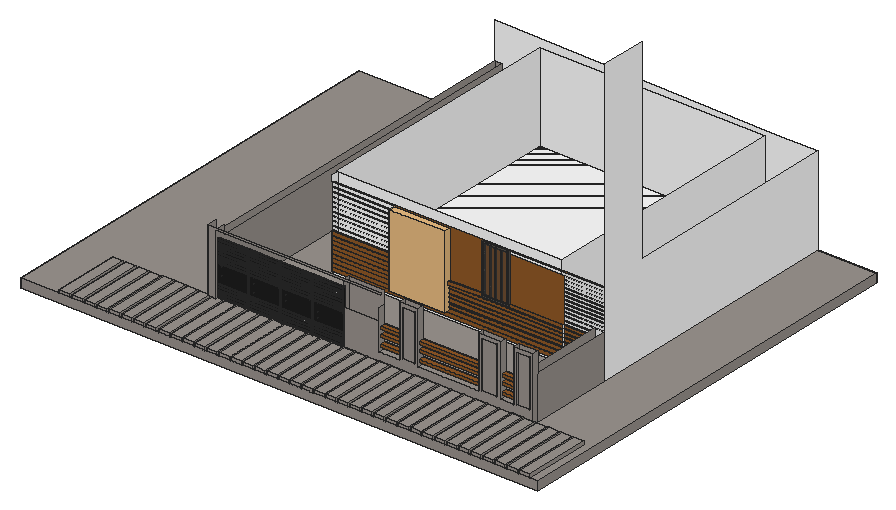
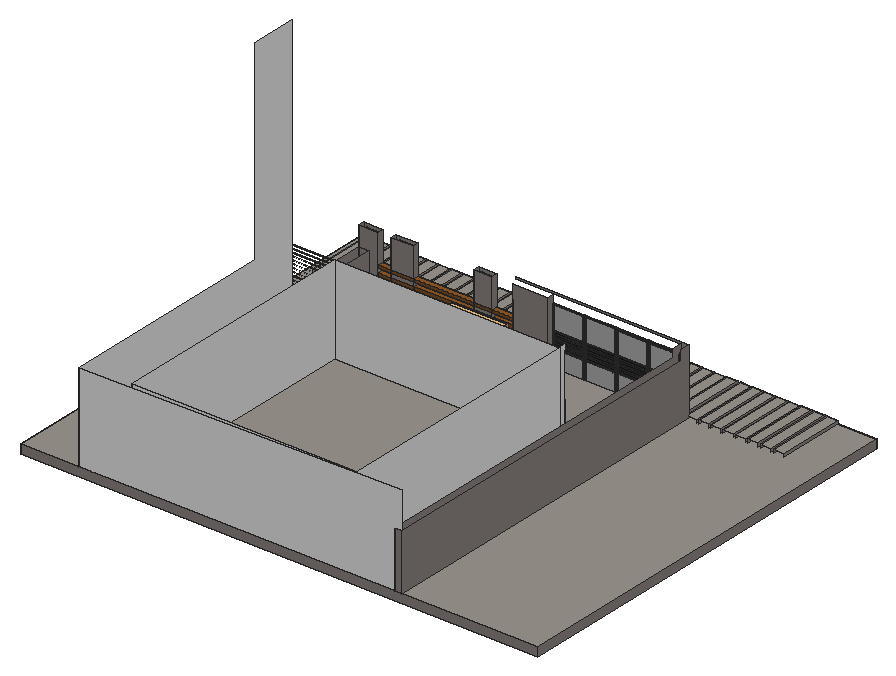
# SketchUp Ruby script. Lengths in inches.
U = 1.inch
M = Sketchup.active_model
def pt(a) = Geom::Point3d.new(a.map { |v| v * U })
def face(e, loops, mat)
  f = e.add_face(loops[0].map { |a| pt(a) })
  loops[1..].each { |l| e.add_face(l.map { |a| pt(a) }).erase! }
  f.material = f.back_material = mat if mat
  f
end
# faces: each face lists its corners as indices into pts; further lists are holes
def faces(e, pts, list, mat = nil) = list.each { |f| face(e, (f[0].is_a?(Array) ? f : [f]).map { |l| l.map { |i| pts[i] } }, mat) }
# xy, xz, yz: faces in a plane at the given z, y or x. An outline is a flat list of corners, or four numbers for a rectangle; further outlines are holes
def ring(l) = l.size == 4 ? [[l[0], l[1]], [l[2], l[1]], [l[2], l[3]], [l[0], l[3]]] : l.each_slice(2).to_a
def flat(e, list, mat, &to3) = list.each { |f| face(e, (f[0].is_a?(Array) ? f : [f]).map { |l| ring(l).map { |u, v| to3.(u, v) } }, mat) }
def xy(e, z, list, mat = nil) = flat(e, list, mat) { |x, y| [x, y, z] }
def xz(e, y, list, mat = nil) = flat(e, list, mat) { |x, z| [x, y, z] }
def yz(e, x, list, mat = nil) = flat(e, list, mat) { |y, z| [x, y, z] }
def lines(e, pts, list) = list.each { |a, b| e.add_line(pt(pts[a]), pt(pts[b])) }
# prism: a flat outline (further loops are holes) pulled along v
def prism(e, loops, v, mat = nil)
  f = face(e, loops, mat); d = Geom::Vector3d.new(v.map { |x| x * U })
  f.pushpull(f.normal.samedirection?(d) ? d.length : -d.length)
end
def box(e, o, s, mat = nil) = prism(e, [[o, [o[0] + s[0], o[1], o[2]], [o[0] + s[0], o[1] + s[1], o[2]], [o[0], o[1] + s[1], o[2]]]], [0, 0, s[2]], mat)
def at(x, y, z, deg = 0) = Geom::Transformation.translation(pt([x, y, z])) * Geom::Transformation.rotation(ORIGIN, Z_AXIS, deg.degrees)
def axes(o, x, y, z) = Geom::Transformation.new([*x, 0, *y, 0, *z, 0, *pt(o).to_a, 1])
def part(name) = M.definitions.add(name)
# library, detail: a bought-in or finely detailed component or shape, given as its bounding box
def library(name, o, s) = part(name).tap { |d| box(d.entities, o, s) }
def detail(e, o, s) = box(e.add_group.entities, o, s)
def put(e, d, t, mat = nil) = e.add_instance(d, t).tap { |i| i.material = mat if mat }
def group(e, t, mat = nil) = e.add_group.tap { |g| g.transformation = t; g.material = mat if mat }.entities
root = M.entities
M.materials.add("Aluminum_Anodized_DarkGray").color = [87, 83, 78]
M.materials.add("Color_008").color = [30, 30, 30]
M.materials.add("Glass_Coated_Black").color = [65, 65, 65]
M.materials["Glass_Coated_Black"].alpha = 0.42
M.materials.add("[0055_LightGoldenrodYellow]").color = [250, 250, 210]
M.materials.add("[0131_Silver]").color = [192, 192, 192]
M.materials.add("[0134_DimGray]").color = [105, 105, 105]
M.materials.add("[Color M00]").color = [255, 255, 255]
M.materials.add("[Granite Tile]").color = [155, 148, 143]
M.materials.add("[Wood Floor Parquet]").color = [145, 89, 39]
c1 = part("Gate slat")
box(c1.entities,[0,0,-2.03],[1.97,0.97,40.94])
c2 = part("Gate frame member")
box(c2.entities,[0,0,0],[1.9,0.97,93.54])
c3 = part("Gate slat \#1")
box(c3.entities,[2.95,0,-2.03],[0.99,0.97,40.94])
c4 = part("Slatted gate leaf")
p = [[42.85,0.97,43.31],[42.85,0.97,44.29]]
lines(c4.entities,p,[[0,1]])
put(c4.entities,c1,axes([3.9375,0,86.61],[0,0,-1],[0,1,0],[1,0,0]),"Color_008")
put(c4.entities,c2,axes([87.6,0,0],[1,0,0],[0,1,0],[0,0,0.92593]),"Color_008")
put(c4.entities,c1,axes([48.6875,0,86.61],[0,0,-1],[0,1,0],[1,0,0]),"Color_008")
put(c4.entities,c2,axes([0,0,0],[1,0,0],[0,1,0],[0,0,0.92593]),"Color_008")
put(c4.entities,c2,axes([42.85,0,0],[1,0,0],[0,1,0],[0,0,0.92593]),"Color_008")
put(c4.entities,c2,axes([44.75,0,0],[1,0,0],[0,1,0],[0,0,0.92593]),"Color_008")
put(c4.entities,c3,axes([3.9375,0,87.11],[0,0,-1],[0,1,0],[1,0,0]),"[0134_DimGray]")
put(c4.entities,c3,axes([48.6875,0,87.11],[0,0,-1],[0,1,0],[1,0,0]),"[0134_DimGray]")
put(c4.entities,c1,axes([48.6875,0,82.68],[0,0,-1],[0,1,0],[1,0,0]),"Color_008")
put(c4.entities,c3,axes([48.6875,0,83.17],[0,0,-1],[0,1,0],[1,0,0]),"[0134_DimGray]")
put(c4.entities,c3,axes([3.9375,0,83.17],[0,0,-1],[0,1,0],[1,0,0]),"[0134_DimGray]")
put(c4.entities,c1,axes([3.9375,0,82.68],[0,0,-1],[0,1,0],[1,0,0]),"Color_008")
put(c4.entities,c3,axes([48.6875,0,75.3],[0,0,-1],[0,1,0],[1,0,0]),"[0134_DimGray]")
put(c4.entities,c1,axes([48.6875,0,78.74],[0,0,-1],[0,1,0],[1,0,0]),"Color_008")
put(c4.entities,c1,axes([48.6875,0,74.8],[0,0,-1],[0,1,0],[1,0,0]),"Color_008")
put(c4.entities,c3,axes([48.6875,0,79.23],[0,0,-1],[0,1,0],[1,0,0]),"[0134_DimGray]")
put(c4.entities,c3,axes([3.9375,0,75.3],[0,0,-1],[0,1,0],[1,0,0]),"[0134_DimGray]")
put(c4.entities,c1,axes([3.9375,0,78.74],[0,0,-1],[0,1,0],[1,0,0]),"Color_008")
put(c4.entities,c3,axes([3.9375,0,79.23],[0,0,-1],[0,1,0],[1,0,0]),"[0134_DimGray]")
put(c4.entities,c1,axes([3.9375,0,74.8],[0,0,-1],[0,1,0],[1,0,0]),"Color_008")
put(c4.entities,c3,axes([48.6875,0,67.42],[0,0,-1],[0,1,0],[1,0,0]),"[0134_DimGray]")
put(c4.entities,c3,axes([3.9375,0,63.48],[0,0,-1],[0,1,0],[1,0,0]),"[0134_DimGray]")
put(c4.entities,c3,axes([48.6875,0,71.36],[0,0,-1],[0,1,0],[1,0,0]),"[0134_DimGray]")
put(c4.entities,c3,axes([3.9375,0,67.42],[0,0,-1],[0,1,0],[1,0,0]),"[0134_DimGray]")
put(c4.entities,c1,axes([3.9375,0,70.87],[0,0,-1],[0,1,0],[1,0,0]),"Color_008")
put(c4.entities,c1,axes([48.6875,0,70.87],[0,0,-1],[0,1,0],[1,0,0]),"Color_008")
put(c4.entities,c1,axes([48.6875,0,66.93],[0,0,-1],[0,1,0],[1,0,0]),"Color_008")
put(c4.entities,c1,axes([48.6875,0,59.06],[0,0,-1],[0,1,0],[1,0,0]),"Color_008")
put(c4.entities,c1,axes([3.9375,0,55.12],[0,0,-1],[0,1,0],[1,0,0]),"Color_008")
put(c4.entities,c1,axes([3.9375,0,62.99],[0,0,-1],[0,1,0],[1,0,0]),"Color_008")
put(c4.entities,c3,axes([3.9375,0,59.55],[0,0,-1],[0,1,0],[1,0,0]),"[0134_DimGray]")
put(c4.entities,c1,axes([3.9375,0,66.93],[0,0,-1],[0,1,0],[1,0,0]),"Color_008")
put(c4.entities,c1,axes([48.6875,0,62.99],[0,0,-1],[0,1,0],[1,0,0]),"Color_008")
put(c4.entities,c3,axes([48.6875,0,59.55],[0,0,-1],[0,1,0],[1,0,0]),"[0134_DimGray]")
put(c4.entities,c3,axes([48.6875,0,63.48],[0,0,-1],[0,1,0],[1,0,0]),"[0134_DimGray]")
put(c4.entities,c1,axes([3.9375,0,59.06],[0,0,-1],[0,1,0],[1,0,0]),"Color_008")
put(c4.entities,c3,axes([3.9375,0,71.36],[0,0,-1],[0,1,0],[1,0,0]),"[0134_DimGray]")
put(c4.entities,c3,axes([3.9375,0,33.96],[0,0,-1],[0,1,0],[1,0,0]),"[0134_DimGray]")
put(c4.entities,c3,axes([48.6875,0,33.96],[0,0,-1],[0,1,0],[1,0,0]),"[0134_DimGray]")
put(c4.entities,c1,axes([3.9375,0,29.53],[0,0,-1],[0,1,0],[1,0,0]),"Color_008")
put(c4.entities,c3,axes([3.9375,0,26.08],[0,0,-1],[0,1,0],[1,0,0]),"[0134_DimGray]")
put(c4.entities,c1,axes([3.9375,0,33.46],[0,0,-1],[0,1,0],[1,0,0]),"Color_008")
put(c4.entities,c1,axes([48.6875,0,29.53],[0,0,-1],[0,1,0],[1,0,0]),"Color_008")
put(c4.entities,c3,axes([48.6875,0,30.02],[0,0,-1],[0,1,0],[1,0,0]),"[0134_DimGray]")
put(c4.entities,c1,axes([3.9375,0,25.59],[0,0,-1],[0,1,0],[1,0,0]),"Color_008")
put(c4.entities,c1,axes([48.6875,0,25.59],[0,0,-1],[0,1,0],[1,0,0]),"Color_008")
put(c4.entities,c1,axes([48.6875,0,33.46],[0,0,-1],[0,1,0],[1,0,0]),"Color_008")
put(c4.entities,c1,axes([3.9375,0,49.7],[0,0,-1],[0,1,0],[1,0,0]),"Color_008")
put(c4.entities,c3,axes([48.6875,0,26.08],[0,0,-1],[0,1,0],[1,0,0]),"[0134_DimGray]")
put(c4.entities,c3,axes([3.9375,0,30.02],[0,0,-1],[0,1,0],[1,0,0]),"[0134_DimGray]")
put(c4.entities,c1,axes([3.9375,0,5.91],[0,0,-1],[0,1,0],[1,0,0]),"Color_008")
put(c4.entities,c1,axes([48.6875,0,13.78],[0,0,-1],[0,1,0],[1,0,0]),"Color_008")
put(c4.entities,c3,axes([48.6875,0,10.33],[0,0,-1],[0,1,0],[1,0,0]),"[0134_DimGray]")
put(c4.entities,c3,axes([3.9375,0,6.4],[0,0,-1],[0,1,0],[1,0,0]),"[0134_DimGray]")
put(c4.entities,c1,axes([3.9375,0,13.78],[0,0,-1],[0,1,0],[1,0,0]),"Color_008")
put(c4.entities,c1,axes([48.6875,0,21.65],[0,0,-1],[0,1,0],[1,0,0]),"Color_008")
put(c4.entities,c1,axes([48.6875,0,5.91],[0,0,-1],[0,1,0],[1,0,0]),"Color_008")
put(c4.entities,c3,axes([48.6875,0,22.15],[0,0,-1],[0,1,0],[1,0,0]),"[0134_DimGray]")
put(c4.entities,c1,axes([48.6875,0,1.97],[0,0,-1],[0,1,0],[1,0,0]),"Color_008")
put(c4.entities,c1,axes([48.6875,0,9.84],[0,0,-1],[0,1,0],[1,0,0]),"Color_008")
put(c4.entities,c3,axes([48.6875,0,6.4],[0,0,-1],[0,1,0],[1,0,0]),"[0134_DimGray]")
put(c4.entities,c1,axes([3.9375,0,9.84],[0,0,-1],[0,1,0],[1,0,0]),"Color_008")
put(c4.entities,c3,axes([3.9375,0,10.33],[0,0,-1],[0,1,0],[1,0,0]),"[0134_DimGray]")
put(c4.entities,c3,axes([3.9375,0,22.15],[0,0,-1],[0,1,0],[1,0,0]),"[0134_DimGray]")
put(c4.entities,c1,axes([3.9375,0,1.97],[0,0,-1],[0,1,0],[1,0,0]),"Color_008")
put(c4.entities,c3,axes([3.9375,0,18.21],[0,0,-1],[0,1,0],[1,0,0]),"[0134_DimGray]")
put(c4.entities,c3,axes([3.9375,0,14.27],[0,0,-1],[0,1,0],[1,0,0]),"[0134_DimGray]")
put(c4.entities,c1,axes([3.9375,0,21.65],[0,0,-1],[0,1,0],[1,0,0]),"Color_008")
put(c4.entities,c3,axes([48.6875,0,18.21],[0,0,-1],[0,1,0],[1,0,0]),"[0134_DimGray]")
put(c4.entities,c1,axes([3.9375,0,17.72],[0,0,-1],[0,1,0],[1,0,0]),"Color_008")
put(c4.entities,c1,axes([48.6875,0,17.72],[0,0,-1],[0,1,0],[1,0,0]),"Color_008")
put(c4.entities,c3,axes([48.6875,0,14.27],[0,0,-1],[0,1,0],[1,0,0]),"[0134_DimGray]")
put(c4.entities,c1,axes([3.9375,0,44.29],[0,0,-1],[0,1,0],[1,0,0]),"Color_008")
put(c4.entities,c1,axes([3.9375,0,38.88],[0,0,-1],[0,1,0],[1,0,0]),"Color_008")
put(c4.entities,c1,axes([48.6875,0,49.7],[0,0,-1],[0,1,0],[1,0,0]),"Color_008")
put(c4.entities,c1,axes([48.6875,0,44.29],[0,0,-1],[0,1,0],[1,0,0]),"Color_008")
put(c4.entities,c1,axes([48.6875,0,38.88],[0,0,-1],[0,1,0],[1,0,0]),"Color_008")
put(c4.entities,c1,axes([48.6875,0,55.12],[0,0,-1],[0,1,0],[1,0,0]),"Color_008")
c5 = part("Gate infill panel \#1")
box(c5.entities,[0,0,-1.97],[52.81,0.39,23.62])
c6 = part("Gate infill panel")
box(c6.entities,[0,0,-9.84],[39.64,0.39,36.58])
c7 = part("Porton casa")
put(c7.entities,c4,axes([13.02,-50.18,0],[0.96774,0,0],[0,1,0],[0,0,1]),"[0055_LightGoldenrodYellow]")
put(c7.entities,c5,axes([13.02,-50.57,33.46],[0.82011,0,0],[0,1,0],[0,0,1]),"Color_008")
put(c7.entities,c6,axes([56.33,-49.21,63.0625],[1.04618,0,0],[0,1,0],[0,0,0.8072]),"[0131_Silver]")
put(c7.entities,c6,axes([56.33,-49.21,9.91],[1.04618,0,0],[0,1,0],[0,0,0.8072]),"[0131_Silver]")
put(c7.entities,c6,axes([14.87,-49.21,9.91],[1.04618,0,0],[0,1,0],[0,0,0.8072]),"[0131_Silver]")
put(c7.entities,c6,axes([14.87,-49.21,63.0625],[1.04618,0,0],[0,1,0],[0,0,0.8072]),"[0131_Silver]")
put(c7.entities,c5,axes([56.33,-50.57,33.46],[0.82011,0,0],[0,1,0],[0,0,1]),"Color_008")
c8 = library("Glass+Door+1800+x+2400",[-92.74,-2.96,0],[74.8,10.14,98.43])
c9 = part("Group\#32")
box(c9.entities,[0,0,0],[182.46,7.0625,3.98])
c10 = part("Untitled")
g1 = group(c10.entities,at(27.48,0,0))
xy(g1,0,[[0,0,54,3]],"Aluminum_Anodized_DarkGray")
xy(g1,2,[[2.25,0,51.75,1],[2.25,2,51.75,3]],"Aluminum_Anodized_DarkGray")
xy(g1,3,[[3.375,1,14.625,1.5],[15.75,1,26.4375,1.5],[27.5625,1,38.25,1.5],[39.375,1,50.625,1.5],[3.375,1.5,14.625,2],
  [15.75,1.5,26.4375,2],[27.5625,1.5,38.25,2],[39.375,1.5,50.625,2]],"Aluminum_Anodized_DarkGray")
xy(g1,99,[[3.375,1,14.625,1.5],[15.75,1,26.4375,1.5],[26.4375,1,27.5625,2],[27.5625,1,38.25,1.5],[38.25,1,39.375,2],
  [39.375,1,50.625,1.5],[3.375,1.5,14.625,2],[15.75,1.5,26.4375,2],[27.5625,1.5,38.25,2],[39.375,1.5,50.625,2]],"Aluminum_Anodized_DarkGray")
xy(g1,100,[[2.25,0,51.75,1],[2.25,2,51.75,3]],"Aluminum_Anodized_DarkGray")
xy(g1,102,[[0,0,54,3]],"Aluminum_Anodized_DarkGray")
xz(g1,0,[[[0,0,54,102],[2.25,2,51.75,100]]],"Aluminum_Anodized_DarkGray")
xz(g1,1,[[[2.25,2,51.75,100],[3.375,3,14.625,99],[39.375,3,50.625,99],[27.5625,3,38.25,99],[15.75,3,26.4375,99]]],"Aluminum_Anodized_DarkGray")
xz(g1,1.5,[[3.375,3,14.625,99],[15.75,3,27,99],[27.5625,3,38.8125,99],[39.375,3,50.625,99]],"Glass_Coated_Black")
xz(g1,2,[[[2.25,2,51.75,100],[3.375,3,14.625,99],[39.375,3,50.625,99],[27.5625,3,38.25,99],[15.75,3,26.4375,99]]],"Aluminum_Anodized_DarkGray")
xz(g1,3,[[[0,0,54,102],[2.25,2,51.75,100]]],"Aluminum_Anodized_DarkGray")
yz(g1,0,[[0,0,3,102]],"Aluminum_Anodized_DarkGray")
yz(g1,2.25,[[0,2,1,100],[2,2,3,100]],"Aluminum_Anodized_DarkGray")
yz(g1,3.375,[[1,3,1.5,99],[1.5,3,2,99]],"Aluminum_Anodized_DarkGray")
yz(g1,14.625,[[1,3,1.5,99],[1.5,3,2,99]],"Aluminum_Anodized_DarkGray")
yz(g1,15.75,[[1,3,1.5,99],[1.5,3,2,99]],"Aluminum_Anodized_DarkGray")
yz(g1,26.4375,[[1,3,2,99]],"Aluminum_Anodized_DarkGray")
yz(g1,27.5625,[[1,3,1.5,99],[1.5,3,2,99]],"Aluminum_Anodized_DarkGray")
yz(g1,38.25,[[1,3,2,99]],"Aluminum_Anodized_DarkGray")
yz(g1,39.375,[[1,3,1.5,99],[1.5,3,2,99]],"Aluminum_Anodized_DarkGray")
yz(g1,50.625,[[1,3,1.5,99],[1.5,3,2,99]],"Aluminum_Anodized_DarkGray")
yz(g1,51.75,[[0,2,1,100],[2,2,3,100]],"Aluminum_Anodized_DarkGray")
yz(g1,54,[[0,0,3,102]],"Aluminum_Anodized_DarkGray")
p = [[15.75,2,99],[14.625,2,99]]
lines(g1,p,[[0,1]])
xy(root,-12,[[607.56,99.5625,620.89,213.625]],"[Granite Tile]")
xy(root,0,[[564.8125,213.625,620.9375,573.625],[251.125,222.625,555.8125,564.625]],"[Color M00]")
xy(root,0,[[365.39,0,379.62,91.25],[183.25,88.8125,193.4375,573.625],[364.82,91.25,620.89,99.5625]],"[Granite Tile]")
xy(root,3.53,[[252.1,212.375,564.8125,213.625]],"[Color M00]")
xy(root,4.3125,[[52.21,0,66.43,91.25],[69.83,0,84.06,91.25],[87.27,0,101.5,91.25],[103.58,0,117.81,91.25],[120.27,0,134.5,91.25],
  [137.21,0,151.43,91.25],[153.21,0,167.43,91.25],[169.89,0,184.12,91.25],[188.14,0,202.37,91.25],[203.96,0,218.18,91.25],
  [220.08,0,234.31,91.25],[236.27,0,250.5,91.25],[252.46,0,266.68,91.25],[269.02,0,283.25,91.25],[285.08,0,299.31,91.25],
  [301.08,0,315.31,91.25],[317.46,0,331.68,91.25],[334.02,0,348.25,91.25],[349.71,0,363.93,91.25],[365.39,0,379.62,91.25],
  [381.52,0,395.75,91.25],[397.71,0,411.93,91.25],[413.58,0,427.81,91.25],[429.64,0,443.87,91.25],[445.71,0,459.93,91.25],
  [461.83,0,476.06,91.25],[478.58,0,492.81,91.25],[495.52,0,509.75,91.25],[511.64,0,525.87,91.25],[528.14,0,542.37,91.25],
  [544.27,0,558.5,91.25],[560.71,0,574.93,91.25],[576.96,0,591.18,91.25],[593.33,0,607.56,91.25],[609.43,0,623.66,91.25],
  [625.74,0,639.97,91.25],[641.99,0,656.22,91.25],[659.37,0,673.59,91.25],[675.55,0,689.78,91.25]],"[Granite Tile]")
xy(root,8.6,[[252.1,212.375,564.8125,213.625]],"[Color M00]")
xy(root,9.03,[[252.1,212.375,564.8125,213.625]],"[Color M00]")
xy(root,14.53,[[252.1,212.375,336.02,213.625]],"[Color M00]")
xy(root,15.65,[[413.01,91.25,440.87,99.5625],[465.26,91.25,547.3,99.5625],[577.46,91.25,595.47,99.5625]],"[Granite Tile]")
xy(root,15.86,[[410.82,212.5,564.8125,213.625]],"[Color M00]")
xy(root,16.1,[[598.93,91.25,617.05,93]],"[Granite Tile]")
xy(root,16.5,[[551.82,91.25,572.14,91.8125]],"[Granite Tile]")
xy(root,17.39,[[444.42,91.25,461.86,91.8125]],"[Granite Tile]")
xy(root,19.6,[[252.1,212.375,336.02,213.625]],"[Color M00]")
xy(root,19.91,[[252.1,212.375,336.02,213.625]],"[Color M00]")
xy(root,20.04,[[410.82,212.5,564.8125,213.625]],"[Color M00]")
xy(root,22.24,[[410.82,212.5,564.8125,213.625]],"[Color M00]")
xy(root,24.97,[[252.1,212.375,336.02,213.625]],"[Color M00]")
xy(root,25.28,[[252.1,212.375,336.02,213.625]],"[Color M00]")
xy(root,26.41,[[410.82,212.5,564.8125,213.625]],"[Color M00]")
xy(root,28.11,[[410.82,212.5,564.8125,213.625]],"[Color M00]")
xy(root,30.35,[[252.1,212.375,336.02,213.625]],"[Color M00]")
xy(root,30.66,[[252.1,212.375,336.02,213.625]],"[Color M00]")
xy(root,32.29,[[410.82,212.5,564.8125,213.625]],"[Color M00]")
xy(root,33.3,[[410.82,212.5,564.8125,213.625]],"[Color M00]")
xy(root,35.72,[[252.1,212.375,336.02,213.625]],"[Color M00]")
xy(root,36.1,[[252.1,212.375,336.02,213.625]],"[Color M00]")
xy(root,37.48,[[410.82,212.5,564.8125,213.625]],"[Color M00]")
xy(root,38.55,[[410.82,212.5,564.8125,213.625]],"[Color M00]")
xy(root,41.16,[[252.1,212.375,336.02,213.625]],"[Color M00]")
xy(root,41.78,[[252.1,212.375,336.02,213.625]],"[Color M00]")
xy(root,42.73,[[410.82,212.5,564.8125,213.625]],"[Color M00]")
xy(root,43.86,[[491.52,212.5,564.8125,213.625]],"[Color M00]")
xy(root,44.55,[[410.51,209.22,410.4,211.4,455.45,213.78,455.57,211.6]],"[Color M00]")
xy(root,46.85,[[252.1,212.375,336.02,213.625]],"[Color M00]")
xy(root,47.6,[[252.1,212.375,336.02,213.625]],"[Color M00]")
xy(root,48.04,[[491.52,212.5,564.8125,213.625]],"[Color M00]")
xy(root,48.79,[[410.51,209.22,455.57,211.6,455.45,213.78,410.4,211.4]],"[Color M00]")
xz(root,0,[[52.21,0,66.43,4.3125],[69.83,0,84.06,4.3125],[87.27,0,101.5,4.3125],[103.58,0,117.81,4.3125],[120.27,0,134.5,4.3125],
  [137.21,0,151.43,4.3125],[153.21,0,167.43,4.3125],[169.89,0,184.12,4.3125],[188.14,0,202.37,4.3125],[203.96,0,218.18,4.3125],
  [220.08,0,234.31,4.3125],[236.27,0,250.5,4.3125],[252.46,0,266.68,4.3125],[269.02,0,283.25,4.3125],[285.08,0,299.31,4.3125],
  [301.08,0,315.31,4.3125],[317.46,0,331.68,4.3125],[334.02,0,348.25,4.3125],[349.71,0,363.93,4.3125],[365.39,0,379.62,4.3125],
  [381.52,0,395.75,4.3125],[397.71,0,411.93,4.3125],[413.58,0,427.81,4.3125],[429.64,0,443.87,4.3125],[445.71,0,459.93,4.3125],
  [461.83,0,476.06,4.3125],[478.58,0,492.81,4.3125],[495.52,0,509.75,4.3125],[511.64,0,525.87,4.3125],[528.14,0,542.37,4.3125],
  [544.27,0,558.5,4.3125],[560.71,0,574.93,4.3125],[576.96,0,591.18,4.3125],[593.33,0,607.56,4.3125],[609.43,0,623.66,4.3125],
  [625.74,0,639.97,4.3125],[641.99,0,656.22,4.3125],[659.37,0,673.59,4.3125],[675.55,0,689.78,4.3125]],"[Granite Tile]")
xz(root,88.8125,[[183.25,0,183.25,89.375,417,89.375,417,86.92,193.4375,86.92,193.4375,0]],"[Granite Tile]")
xz(root,91.25,[[[364.82,0,365.39,0,365.39,4.3125,379.62,4.3125,379.62,0,381.52,0,381.52,4.3125,395.75,4.3125,395.75,0,397.71,0,397.71,4.3125,411.93,4.3125,411.93,0,413.58,0,413.58,4.3125,427.81,4.3125,427.81,0,429.64,0,429.64,4.3125,443.87,4.3125,443.87,0,445.71,0,445.71,4.3125,459.93,4.3125,459.93,0,461.83,0,461.83,4.3125,476.06,4.3125,476.06,0,478.58,0,478.58,4.3125,492.81,4.3125,492.81,0,495.52,0,495.52,4.3125,509.75,4.3125,509.75,0,511.64,0,511.64,4.3125,525.87,4.3125,525.87,0,528.14,0,528.14,4.3125,542.37,4.3125,542.37,0,544.27,0,544.27,4.3125,558.5,4.3125,558.5,0,560.71,0,560.71,4.3125,574.93,4.3125,574.93,0,576.96,0,576.96,4.3125,591.18,4.3125,591.18,0,593.33,0,593.33,4.3125,607.56,4.3125,607.56,0,609.43,0,609.43,4.3125,620.89,4.3125,620.89,85.375,595.47,85.375,595.47,15.65,577.46,15.65,577.46,85.375,547.3,85.375,547.3,15.65,465.26,15.65,465.26,85.375,440.87,85.375,440.87,15.65,413.01,15.65,413.01,52.49,364.82,52.49],[551.82,16.5,572.14,80.75],[598.93,16.1,617.05,80.85],[444.42,17.39,461.86,80.89]],[365.39,0,379.62,4.3125],[381.52,0,395.75,4.3125],[397.71,0,411.93,4.3125],[413.58,0,427.81,4.3125],
  [429.64,0,443.87,4.3125],[445.71,0,459.93,4.3125],[461.83,0,476.06,4.3125],[478.58,0,492.81,4.3125],[495.52,0,509.75,4.3125],
  [511.64,0,525.87,4.3125],[528.14,0,542.37,4.3125],[544.27,0,558.5,4.3125],[560.71,0,574.93,4.3125],[576.96,0,591.18,4.3125],
  [593.33,0,607.56,4.3125],[609.43,0,620.89,4.3125]],"[Granite Tile]")
xz(root,91.8125,[[551.82,16.5,572.14,80.75],[444.42,17.39,461.86,80.89]],"[Granite Tile]")
xz(root,93,[[598.93,16.1,617.05,80.85]],"[Granite Tile]")
xz(root,99.5625,[[607.56,-12,620.89,0],[364.82,0,364.82,86.9375,413.01,86.9375,413.01,15.65,440.87,15.65,440.87,85.375,465.26,85.375,465.26,15.65,547.3,15.65,547.3,85.375,577.46,85.375,577.46,15.65,595.47,15.65,595.47,85.375,620.89,85.375,620.89,58.6875,607.56,58.6875,607.56,0],[607.56,0,620.89,58.6875]],"[Granite Tile]")
xz(root,212.375,[[252.1,3.53,564.8125,8.6],[252.1,9.03,564.8125,14.1],[252.1,14.53,336.02,19.6],[252.1,19.91,336.02,24.97],[252.1,25.28,336.02,30.35],
  [252.1,30.66,336.02,35.72],[252.1,36.1,336.02,41.16],[252.1,41.78,336.02,46.85],[252.1,47.6,336.02,52.66]],"[Wood Floor Parquet]")
xz(root,212.5,[[410.82,15.86,564.8125,20.04],[410.82,22.24,564.8125,26.41],[410.82,28.11,564.8125,32.29],[410.82,33.3,564.8125,37.48],[410.82,38.55,564.8125,42.73],
  [491.52,43.86,564.8125,48.04]],"[Wood Floor Parquet]")
xz(root,213.625,[[252.1,0,607.56,3.53],[607.56,0,620.89,3.53],[620.89,0,620.9375,3.53],[252.1,3.53,564.8125,8.6],[252.1,8.6,607.56,9.03],
  [607.56,8.6,620.89,9.03],[620.89,8.6,620.9375,9.03],[252.1,14.53,336.02,19.6],[410.82,15.86,564.8125,20.04],[252.1,19.91,336.02,24.97],
  [410.82,22.24,564.8125,26.41],[252.1,25.28,336.02,30.35],[410.82,28.11,564.8125,32.29],[252.1,30.66,336.02,35.72],[410.82,33.3,564.8125,37.48],
  [252.1,36.1,336.02,41.16],[410.82,38.55,564.8125,42.73],[252.1,41.78,336.02,46.85],[252.1,47.6,336.02,52.66]],"[Color M00]")
xz(root,213.625,[[607.56,-12,620.89,0]],"[Granite Tile]")
xz(root,213.625,[[564.8125,3.53,607.56,8.6],[607.56,3.53,620.89,8.6],[620.89,3.53,620.9375,8.6],[252.1,9.03,564.8125,9.03,564.8125,14.1,607.56,14.1,607.56,15.86,410.82,15.86,410.82,20.04,607.56,20.04,607.56,22.24,410.82,22.24,410.82,26.41,607.56,26.41,607.56,28.11,410.82,28.11,410.82,32.29,607.56,32.29,607.56,33.3,410.82,33.3,410.82,37.48,607.56,37.48,607.56,38.55,410.82,38.55,410.82,42.73,607.56,42.73,607.56,43.86,564.8125,43.86,564.8125,48.04,607.56,48.04,607.56,48.99,564.8125,48.99,564.8125,53.16,607.56,53.16,607.56,54.18,564.8125,54.18,564.8125,58.35,620.9375,58.35,620.9375,59.36,564.8125,59.36,564.8125,63.54,620.9375,63.54,620.9375,64.36,564.8125,64.36,564.8125,68.54,620.9375,68.54,620.9375,69.36,564.8125,69.36,564.8125,73.54,620.9375,73.54,620.9375,74.43,564.8125,74.43,564.8125,78.6,620.9375,78.6,620.9375,79.18,564.8125,79.18,564.8125,83.35,620.9375,83.35,620.9375,83.93,564.8125,83.93,564.8125,88.1,620.9375,88.1,620.9375,88.68,564.8125,88.68,564.8125,92.85,620.9375,92.85,620.9375,93.36,564.8125,93.36,564.8125,97.54,620.9375,97.54,620.9375,97.99,564.8125,97.99,564.8125,102.16,620.9375,102.16,620.9375,102.82,564.8125,102.82,564.8125,106.99,620.9375,106.99,620.9375,107.57,491.52,107.57,491.52,111.74,620.9375,111.74,620.9375,113.1,252.1,113.1,252.1,111.2,336.02,111.2,336.02,106.14,252.1,106.14,252.1,104.89,336.02,104.89,336.02,99.83,252.1,99.83,252.1,98.7,336.02,98.7,336.02,93.64,252.1,93.64,252.1,92.64,336.02,92.64,336.02,87.58,252.1,87.58,252.1,86.53,336.02,86.53,336.02,81.47,252.1,81.47,252.1,80.85,336.02,80.85,336.02,75.78,252.1,75.78,252.1,75.35,336.02,75.35,336.02,70.28,252.1,70.28,252.1,69.66,336.02,69.66,336.02,64.6,252.1,64.6,252.1,63.97,336.02,63.97,336.02,58.91,252.1,58.91,252.1,58.41,336.02,58.41,336.02,53.35,252.1,53.35,252.1,52.66,336.02,52.66,336.02,47.6,252.1,47.6,252.1,46.85,336.02,46.85,336.02,41.78,252.1,41.78,252.1,41.16,336.02,41.16,336.02,36.1,252.1,36.1,252.1,35.72,336.02,35.72,336.02,30.66,252.1,30.66,252.1,30.35,336.02,30.35,336.02,25.28,252.1,25.28,252.1,24.97,336.02,24.97,336.02,19.91,252.1,19.91,252.1,19.6,336.02,19.6,336.02,14.53,252.1,14.53],[564.8125,9.03,607.56,14.1],
  [607.56,9.03,620.89,14.1],[620.89,9.03,620.9375,14.1],[607.56,14.1,620.89,15.86],[620.89,14.1,620.9375,15.86],[564.8125,15.86,607.56,20.04],
  [607.56,15.86,620.89,20.04],[620.89,15.86,620.9375,20.04],[607.56,20.04,620.89,22.24],[620.89,20.04,620.9375,22.24],[564.8125,22.24,607.56,26.41],
  [607.56,22.24,620.89,26.41],[620.89,22.24,620.9375,26.41],[607.56,26.41,620.89,28.11],[620.89,26.41,620.9375,28.11],[564.8125,28.11,607.56,32.29],
  [607.56,28.11,620.89,32.29],[620.89,28.11,620.9375,32.29],[607.56,32.29,620.89,33.3],[620.89,32.29,620.9375,33.3],[564.8125,33.3,607.56,37.48],
  [607.56,33.3,620.89,37.48],[620.89,33.3,620.9375,37.48],[607.56,37.48,620.89,38.55],[620.89,37.48,620.9375,38.55],[564.8125,38.55,607.56,42.73],
  [607.56,38.55,620.89,42.73],[620.89,38.55,620.9375,42.73],[607.56,42.73,620.89,43.86],[620.89,42.73,620.9375,43.86],[564.8125,43.86,607.56,48.04],
  [607.56,43.86,620.89,48.04],[620.89,43.86,620.9375,48.04],[607.56,48.04,620.89,48.99],[620.89,48.04,620.9375,48.99]],"[Wood Floor Parquet]")
xz(root,222.625,[[251.125,0,252.1,120],[252.1,0,555.8125,120]],"[Color M00]")
xz(root,564.625,[[251.125,0,555.8125,120]],"[Color M00]")
xz(root,573.625,[[193.4375,0,193.4375,75.6875,183.25,75.6875,183.25,125.32,564.8125,120,620.9375,120,620.9375,0]],"[Color M00]")
xz(root,573.625,[[183.25,0,193.4375,75.6875]],"[Granite Tile]")
yz(root,52.21,[[0,0,91.25,4.3125]],"[Granite Tile]")
yz(root,66.43,[[0,0,91.25,4.3125]],"[Granite Tile]")
yz(root,69.83,[[0,0,91.25,4.3125]],"[Granite Tile]")
yz(root,84.06,[[0,0,91.25,4.3125]],"[Granite Tile]")
yz(root,87.27,[[0,0,91.25,4.3125]],"[Granite Tile]")
yz(root,101.5,[[0,0,91.25,4.3125]],"[Granite Tile]")
yz(root,103.58,[[0,0,91.25,4.3125]],"[Granite Tile]")
yz(root,117.81,[[0,0,91.25,4.3125]],"[Granite Tile]")
yz(root,120.27,[[0,0,91.25,4.3125]],"[Granite Tile]")
yz(root,134.5,[[0,0,91.25,4.3125]],"[Granite Tile]")
yz(root,137.21,[[0,0,91.25,4.3125]],"[Granite Tile]")
yz(root,151.43,[[0,0,91.25,4.3125]],"[Granite Tile]")
yz(root,153.21,[[0,0,91.25,4.3125]],"[Granite Tile]")
yz(root,167.43,[[0,0,91.25,4.3125]],"[Granite Tile]")
yz(root,169.89,[[0,0,91.25,4.3125]],"[Granite Tile]")
yz(root,183.25,[[88.8125,0,573.625,0,573.625,75.6875,102.22,75.6875,102.22,89.375,88.8125,89.375]],"[Granite Tile]")
yz(root,184.12,[[0,0,91.25,4.3125]],"[Granite Tile]")
yz(root,188.14,[[0,0,91.25,4.3125]],"[Granite Tile]")
yz(root,193.4375,[[88.8125,0,88.8125,86.92,102.22,86.92,102.22,75.6875,573.625,75.6875,573.625,0]],"[Granite Tile]")
yz(root,202.37,[[0,0,91.25,4.3125]],"[Granite Tile]")
yz(root,203.96,[[0,0,91.25,4.3125]],"[Granite Tile]")
yz(root,218.18,[[0,0,91.25,4.3125]],"[Granite Tile]")
yz(root,220.08,[[0,0,91.25,4.3125]],"[Granite Tile]")
yz(root,234.31,[[0,0,91.25,4.3125]],"[Granite Tile]")
yz(root,236.27,[[0,0,91.25,4.3125]],"[Granite Tile]")
yz(root,250.5,[[0,0,91.25,4.3125]],"[Granite Tile]")
yz(root,251.125,[[222.625,0,564.625,120]],"[Color M00]")
yz(root,252.1,[[213.625,0,213.625,113.1,212.5,113.1,212.5,120,222.625,120,222.625,0],[212.375,3.53,213.625,8.6],[212.375,9.03,213.625,14.1],[212.375,14.53,213.625,19.6],[212.375,19.91,213.625,24.97],
  [212.375,25.28,213.625,30.35],[212.375,30.66,213.625,35.72],[212.375,36.1,213.625,41.16],[212.375,41.78,213.625,46.85],[212.375,47.6,213.625,52.66]],"[Color M00]")
yz(root,252.46,[[0,0,91.25,4.3125]],"[Granite Tile]")
yz(root,266.68,[[0,0,91.25,4.3125]],"[Granite Tile]")
yz(root,269.02,[[0,0,91.25,4.3125]],"[Granite Tile]")
yz(root,283.25,[[0,0,91.25,4.3125]],"[Granite Tile]")
yz(root,285.08,[[0,0,91.25,4.3125]],"[Granite Tile]")
yz(root,299.31,[[0,0,91.25,4.3125]],"[Granite Tile]")
yz(root,301.08,[[0,0,91.25,4.3125]],"[Granite Tile]")
yz(root,315.31,[[0,0,91.25,4.3125]],"[Granite Tile]")
yz(root,317.46,[[0,0,91.25,4.3125]],"[Granite Tile]")
yz(root,331.68,[[0,0,91.25,4.3125]],"[Granite Tile]")
yz(root,334.02,[[0,0,91.25,4.3125]],"[Granite Tile]")
yz(root,336.02,[[212.375,14.53,213.625,19.6],[212.375,19.91,213.625,24.97],[212.375,25.28,213.625,30.35],[212.375,30.66,213.625,35.72],[212.375,36.1,213.625,41.16],
  [212.375,41.78,213.625,46.85],[212.375,47.6,213.625,52.66]],"[Color M00]")
yz(root,348.25,[[0,0,91.25,4.3125]],"[Granite Tile]")
yz(root,349.71,[[0,0,91.25,4.3125]],"[Granite Tile]")
yz(root,363.93,[[0,0,91.25,4.3125]],"[Granite Tile]")
yz(root,364.82,[[91.25,0,99.5625,86.9375]],"[Granite Tile]")
yz(root,365.39,[[0,0,91.25,4.3125]],"[Granite Tile]")
yz(root,379.62,[[0,0,91.25,4.3125]],"[Granite Tile]")
yz(root,381.52,[[0,0,91.25,4.3125]],"[Granite Tile]")
yz(root,395.75,[[0,0,91.25,4.3125]],"[Granite Tile]")
yz(root,397.71,[[0,0,91.25,4.3125]],"[Granite Tile]")
yz(root,410.82,[[212.5,15.86,213.625,20.04],[212.5,22.24,213.625,26.41],[212.5,28.11,213.625,32.29],[212.5,33.3,213.625,37.48],[212.5,38.55,213.625,42.73]],"[Color M00]")
yz(root,411.93,[[0,0,91.25,4.3125]],"[Granite Tile]")
yz(root,413.01,[[91.25,15.65,99.5625,68.63]],"[Granite Tile]")
yz(root,413.58,[[0,0,91.25,4.3125]],"[Granite Tile]")
yz(root,427.81,[[0,0,91.25,4.3125]],"[Granite Tile]")
yz(root,429.64,[[0,0,91.25,4.3125]],"[Granite Tile]")
yz(root,440.87,[[91.25,15.65,99.5625,85.375]],"[Granite Tile]")
yz(root,443.87,[[0,0,91.25,4.3125]],"[Granite Tile]")
yz(root,444.42,[[91.25,17.39,91.8125,80.89]],"[Granite Tile]")
yz(root,445.71,[[0,0,91.25,4.3125]],"[Granite Tile]")
yz(root,459.93,[[0,0,91.25,4.3125]],"[Granite Tile]")
yz(root,461.83,[[0,0,91.25,4.3125]],"[Granite Tile]")
yz(root,461.86,[[91.25,17.39,91.8125,80.89]],"[Granite Tile]")
yz(root,465.26,[[91.25,15.65,99.5625,85.375]],"[Granite Tile]")
yz(root,476.06,[[0,0,91.25,4.3125]],"[Granite Tile]")
yz(root,478.58,[[0,0,91.25,4.3125]],"[Granite Tile]")
yz(root,492.81,[[0,0,91.25,4.3125]],"[Granite Tile]")
yz(root,495.52,[[0,0,91.25,4.3125]],"[Granite Tile]")
yz(root,509.75,[[0,0,91.25,4.3125]],"[Granite Tile]")
yz(root,511.64,[[0,0,91.25,4.3125]],"[Granite Tile]")
yz(root,525.87,[[0,0,91.25,4.3125]],"[Granite Tile]")
yz(root,528.14,[[0,0,91.25,4.3125]],"[Granite Tile]")
yz(root,542.37,[[0,0,91.25,4.3125]],"[Granite Tile]")
yz(root,544.27,[[0,0,91.25,4.3125]],"[Granite Tile]")
yz(root,547.3,[[91.25,15.65,99.5625,85.375]],"[Granite Tile]")
yz(root,551.82,[[91.25,16.5,91.8125,80.75]],"[Granite Tile]")
yz(root,555.8125,[[222.625,0,564.625,120]],"[Color M00]")
yz(root,558.5,[[0,0,91.25,4.3125]],"[Granite Tile]")
yz(root,560.71,[[0,0,91.25,4.3125]],"[Granite Tile]")
yz(root,564.8125,[[212.375,3.53,213.625,8.6],[212.375,9.03,213.625,14.1],[212.5,15.86,213.625,20.04],[212.5,22.24,213.625,26.41],[212.5,28.11,213.625,32.29],
  [212.5,33.3,213.625,37.48],[212.5,38.55,213.625,42.73],[212.5,43.86,213.625,48.04]],"[Color M00]")
yz(root,572.14,[[91.25,16.5,91.8125,80.75]],"[Granite Tile]")
yz(root,574.93,[[0,0,91.25,4.3125]],"[Granite Tile]")
yz(root,576.96,[[0,0,91.25,4.3125]],"[Granite Tile]")
yz(root,577.46,[[91.25,15.65,99.5625,85.375]],"[Granite Tile]")
yz(root,591.18,[[0,0,91.25,4.3125]],"[Granite Tile]")
yz(root,593.33,[[0,0,91.25,4.3125]],"[Granite Tile]")
yz(root,595.47,[[91.25,15.65,99.5625,85.375]],"[Granite Tile]")
yz(root,598.93,[[91.25,16.1,93,80.85]],"[Granite Tile]")
yz(root,607.56,[[99.5625,-12,213.625,58.6875],[0,0,91.25,4.3125]],"[Granite Tile]")
yz(root,609.43,[[0,0,91.25,4.3125]],"[Granite Tile]")
yz(root,617.05,[[91.25,16.1,93,80.85]],"[Granite Tile]")
yz(root,620.89,[[99.5625,-12,213.625,58.6875],[91.25,0,99.5625,85.375]],"[Granite Tile]")
yz(root,620.9375,[[213.625,0,573.625,0,573.625,120,275.23,120,275.23,384,213.625,384,213.625,120,212.5,120,212.5,113.1,213.625,113.1]],"[Color M00]")
yz(root,623.66,[[0,0,91.25,4.3125]],"[Granite Tile]")
yz(root,625.74,[[0,0,91.25,4.3125]],"[Granite Tile]")
yz(root,639.97,[[0,0,91.25,4.3125]],"[Granite Tile]")
yz(root,641.99,[[0,0,91.25,4.3125]],"[Granite Tile]")
yz(root,656.22,[[0,0,91.25,4.3125]],"[Granite Tile]")
yz(root,659.37,[[0,0,91.25,4.3125]],"[Granite Tile]")
yz(root,673.59,[[0,0,91.25,4.3125]],"[Granite Tile]")
yz(root,675.55,[[0,0,91.25,4.3125]],"[Granite Tile]")
yz(root,689.78,[[0,0,91.25,4.3125]],"[Granite Tile]")
p = [[410.51,209.22,44.55],[455.57,211.6,44.55],[455.57,211.6,48.79],[410.51,209.22,48.79],[410.4,211.4,39.93],[410.51,209.22,39.93],
  [410.4,211.4,44.16],[410.51,209.22,44.16],[410.4,211.4,39.29],[410.51,209.22,39.29],[410.4,211.4,35.05],[410.51,209.22,35.05],
  [410.07,211.39,30.36],[410.18,209.2,30.36],[410.07,211.39,34.6],[410.18,209.2,34.6],[410.07,211.39,25.36],[410.18,209.2,25.36],
  [410.07,211.39,29.6],[410.18,209.2,29.6],[410.07,211.39,19.92],[410.18,209.2,19.92],[410.07,211.39,24.16],[410.18,209.2,24.16],
  [410.07,211.39,18.78],[410.18,209.2,18.78],[410.07,211.39,14.54],[410.18,209.2,14.54],[455.24,211.58,14.52],[455.24,211.58,14.54],
  [491.52,213.625,37.6],[491.52,213.625,37.48]]
faces(root,p,[[0,1,2,3]],"[Wood Floor Parquet]")
lines(root,p,[[4,5],[6,7],[5,7],[8,9],[10,11],[11,9],[12,13],[14,15],[13,15],[16,17],[18,19],[17,19],
  [20,21],[22,23],[21,23],[24,25],[26,27],[27,25],[28,29],[30,31]])
g2 = group(root,at(204.8125,573.625,-12),"[Granite Tile]")
box(g2,[-204.8125,-573.625,0],[700.25,573.625,12])
put(root,c7,at(178.57,141.71,-9.05),"[Granite Tile]")
put(root,c7,at(265.1875,141.71,-9.05),"[Granite Tile]")
put(root,c8,at(428.76,207.49,12.69),"[Color M00]")
put(root,c9,at(413.01,92.5,20.69),"[Wood Floor Parquet]")
put(root,c9,at(413.01,92.5,32.69),"[Wood Floor Parquet]")
put(root,c9,at(413.01,92.5,42.32),"[Wood Floor Parquet]")
put(root,c10,axes([437.75,211.64,44.76],[0.66,0,0],[0,0.66,0],[0,0,0.66]),"[Color M00]")
